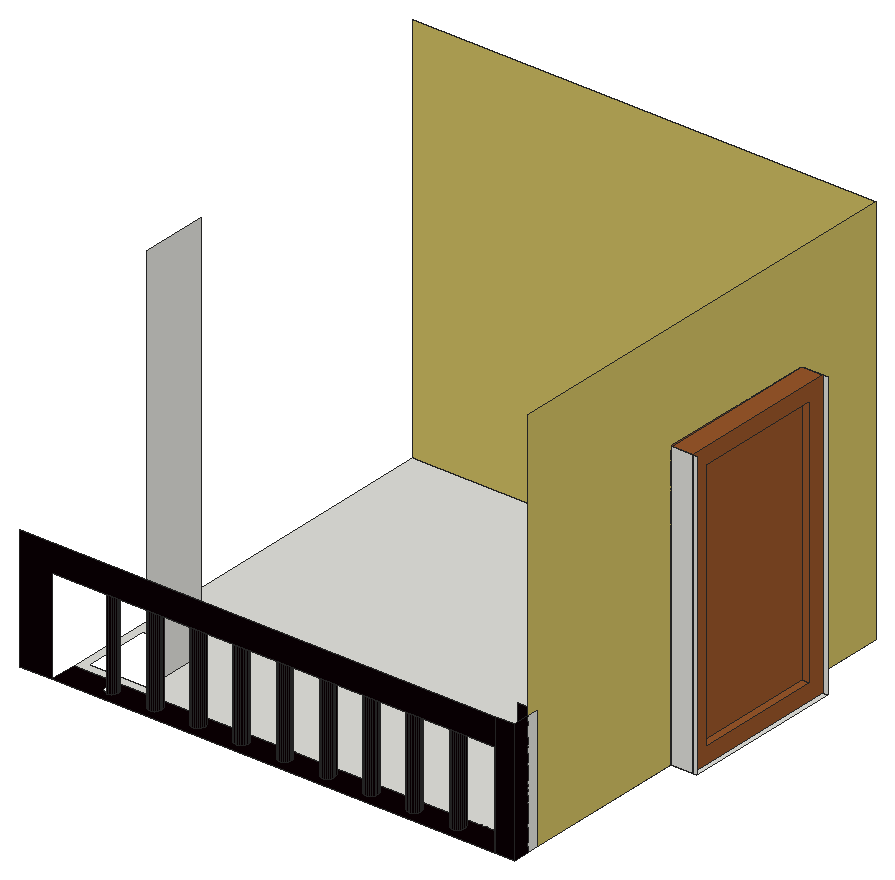
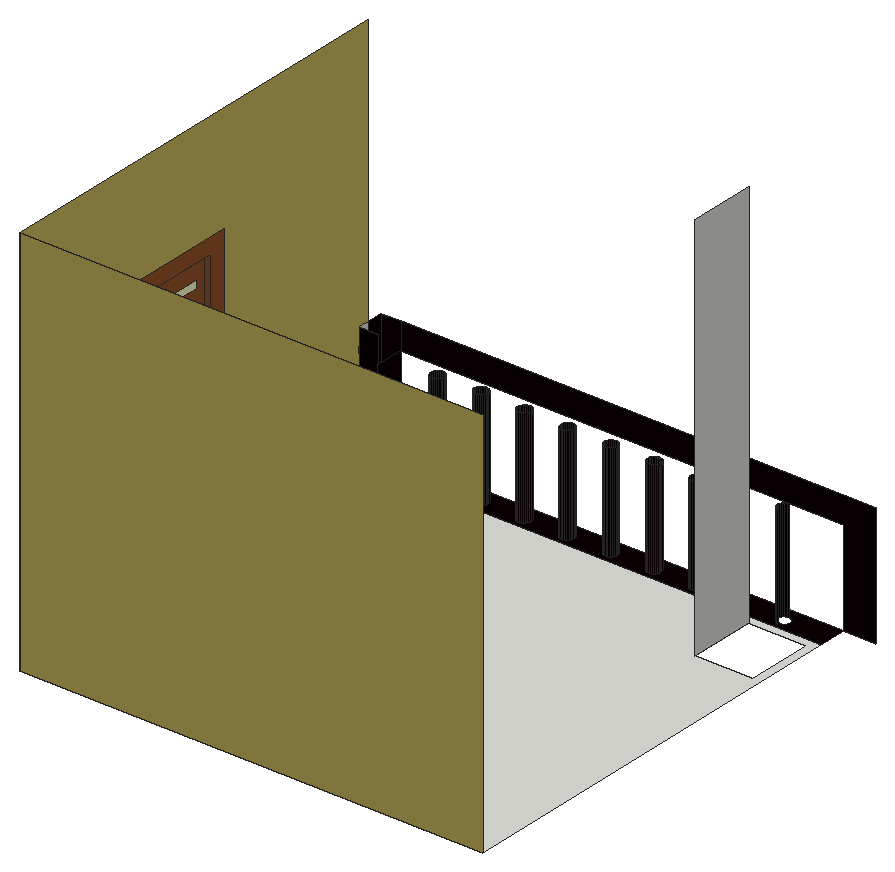
# SketchUp Ruby script. Lengths in inches.
U = 1.inch
M = Sketchup.active_model
def pt(a) = Geom::Point3d.new(a.map { |v| v * U })
def face(e, loops, mat)
  f = e.add_face(loops[0].map { |a| pt(a) })
  loops[1..].each { |l| e.add_face(l.map { |a| pt(a) }).erase! }
  f.material = f.back_material = mat if mat
  f
end
# faces: each face lists its corners as indices into pts; further lists are holes
def faces(e, pts, list, mat = nil) = list.each { |f| face(e, (f[0].is_a?(Array) ? f : [f]).map { |l| l.map { |i| pts[i] } }, mat) }
# xy, xz, yz: faces in a plane at the given z, y or x. An outline is a flat list of corners, or four numbers for a rectangle; further outlines are holes
def ring(l) = l.size == 4 ? [[l[0], l[1]], [l[2], l[1]], [l[2], l[3]], [l[0], l[3]]] : l.each_slice(2).to_a
def flat(e, list, mat, &to3) = list.each { |f| face(e, (f[0].is_a?(Array) ? f : [f]).map { |l| ring(l).map { |u, v| to3.(u, v) } }, mat) }
def xy(e, z, list, mat = nil) = flat(e, list, mat) { |x, y| [x, y, z] }
def xz(e, y, list, mat = nil) = flat(e, list, mat) { |x, z| [x, y, z] }
def yz(e, x, list, mat = nil) = flat(e, list, mat) { |y, z| [x, y, z] }
def lines(e, pts, list) = list.each { |a, b| e.add_line(pt(pts[a]), pt(pts[b])) }
# prism: a flat outline (further loops are holes) pulled along v
def prism(e, loops, v, mat = nil)
  f = face(e, loops, mat); d = Geom::Vector3d.new(v.map { |x| x * U })
  f.pushpull(f.normal.samedirection?(d) ? d.length : -d.length)
end
def box(e, o, s, mat = nil) = prism(e, [[o, [o[0] + s[0], o[1], o[2]], [o[0] + s[0], o[1] + s[1], o[2]], [o[0], o[1] + s[1], o[2]]]], [0, 0, s[2]], mat)
def at(x, y, z, deg = 0) = Geom::Transformation.translation(pt([x, y, z])) * Geom::Transformation.rotation(ORIGIN, Z_AXIS, deg.degrees)
def axes(o, x, y, z) = Geom::Transformation.new([*x, 0, *y, 0, *z, 0, *pt(o).to_a, 1])
def part(name) = M.definitions.add(name)
# library, detail: a bought-in or finely detailed component or shape, given as its bounding box
def library(name, o, s) = part(name).tap { |d| box(d.entities, o, s) }
def detail(e, o, s) = box(e.add_group.entities, o, s)
def put(e, d, t, mat = nil) = e.add_instance(d, t).tap { |i| i.material = mat if mat }
def group(e, t, mat = nil) = e.add_group.tap { |g| g.transformation = t; g.material = mat if mat }.entities
root = M.entities
M.materials.add("[Color D05]").color = [208, 191, 99]
M.materials.add("[Color E01]").color = [255, 255, 204]
M.materials.add("[Metal Seamed]").color = [11, 0, 4]
M.materials.add("[Wood Cherry Original]").color = [152, 86, 42]
c1 = part("Group\#1")
xy(c1.entities,0,[[0,0,6.3125,48]],"[Wood Cherry Original]")
xy(c1.entities,4.83,[[2.3125,4.83,3.9375,43.17]])
xy(c1.entities,4.83,[[0,4.83,2.3125,43.17],[3.9375,4.83,6.3125,43.17]],"[Wood Cherry Original]")
xy(c1.entities,79.17,[[2.3125,4.83,3.9375,43.17]])
xy(c1.entities,79.17,[[0,4.83,2.3125,43.17],[3.9375,4.83,6.3125,43.17]],"[Wood Cherry Original]")
xy(c1.entities,84,[[0,0,6.3125,48]],"[Wood Cherry Original]")
xz(c1.entities,0,[[0,0,6.3125,84]],"[Wood Cherry Original]")
xz(c1.entities,4.83,[[2.3125,4.83,3.9375,79.17]])
xz(c1.entities,4.83,[[0,4.83,2.3125,79.17],[3.9375,4.83,6.3125,79.17]],"[Wood Cherry Original]")
xz(c1.entities,43.17,[[2.3125,4.83,3.9375,79.17]])
xz(c1.entities,43.17,[[0,4.83,2.3125,79.17],[3.9375,4.83,6.3125,79.17]],"[Wood Cherry Original]")
xz(c1.entities,48,[[0,0,6.3125,84]],"[Wood Cherry Original]")
yz(c1.entities,0,[[[0,0,48,84],[4.83,4.83,43.17,79.17]]],"[Wood Cherry Original]")
yz(c1.entities,2.3125,[[7.68,9.76,40.37,11.76],[7.68,18.32,40.37,20.32],[7.68,27.01,40.37,29.01],[7.68,35.69,40.37,37.69],[7.68,44.38,40.37,46.38],
  [7.68,53.07,40.37,55.07],[7.68,61.76,40.37,63.76],[7.68,70.44,40.37,72.44]],"[Color E01]")
yz(c1.entities,2.3125,[[[4.83,4.83,43.17,79.17],[7.68,70.44,40.37,72.44],[7.68,61.76,40.37,63.76],[7.68,53.07,40.37,55.07],[7.68,44.38,40.37,46.38],[7.68,35.69,40.37,37.69],[7.68,27.01,40.37,29.01],[7.68,18.32,40.37,20.32],[7.68,9.76,40.37,11.76]]],"[Wood Cherry Original]")
yz(c1.entities,3.9375,[[4.83,4.83,43.17,79.17]],"[Wood Cherry Original]")
yz(c1.entities,6.3125,[[[0,0,48,84],[4.83,4.83,43.17,79.17]]],"[Wood Cherry Original]")
xy(root,148.4375,[[152.3,62.41,158,70.73],[48.66,65.07,48.15,65.08,47.67,65.22,47.23,65.48,46.88,65.84,46.64,66.29,46.51,66.78,46.52,67.28,46.66,67.77,46.92,68.2,47.28,68.55,47.73,68.8,48.22,68.92,48.72,68.91,49.21,68.78,49.64,68.52,50,68.15,50.24,67.71,50.36,67.22,50.36,66.71,50.22,66.23,49.96,65.79,49.59,65.44,49.15,65.2],[61.41,65.07,60.9,65.08,60.42,65.22,59.98,65.48,59.63,65.84,59.39,66.29,59.26,66.78,59.27,67.28,59.41,67.77,59.67,68.2,60.03,68.55,60.48,68.8,60.97,68.92,61.47,68.91,61.96,68.78,62.39,68.52,62.75,68.15,62.99,67.71,63.11,67.22,63.11,66.71,62.97,66.23,62.71,65.79,62.34,65.44,61.9,65.2],[74.16,65.07,73.65,65.08,73.17,65.22,72.73,65.48,72.38,65.84,72.14,66.29,72.01,66.78,72.02,67.28,72.16,67.77,72.42,68.2,72.78,68.55,73.23,68.8,73.72,68.92,74.22,68.91,74.71,68.78,75.14,68.52,75.5,68.15,75.74,67.71,75.86,67.22,75.86,66.71,75.72,66.23,75.46,65.79,75.09,65.44,74.65,65.2],[86.91,65.07,86.4,65.08,85.92,65.22,85.48,65.48,85.13,65.84,84.89,66.29,84.76,66.78,84.77,67.28,84.91,67.77,85.17,68.2,85.53,68.55,85.98,68.8,86.47,68.92,86.97,68.91,87.46,68.78,87.89,68.52,88.25,68.15,88.49,67.71,88.61,67.22,88.61,66.71,88.47,66.23,88.21,65.79,87.84,65.44,87.4,65.2],
  [99.66,65.07,99.15,65.08,98.67,65.22,98.23,65.48,97.88,65.84,97.64,66.29,97.51,66.78,97.52,67.28,97.66,67.77,97.92,68.2,98.28,68.55,98.73,68.8,99.22,68.92,99.72,68.91,100.21,68.78,100.64,68.52,101,68.15,101.24,67.71,101.36,67.22,101.36,66.71,101.22,66.23,100.96,65.79,100.59,65.44,100.15,65.2],[112.41,65.07,111.9,65.08,111.42,65.22,110.98,65.48,110.63,65.84,110.39,66.29,110.26,66.78,110.27,67.28,110.41,67.77,110.67,68.2,111.03,68.55,111.48,68.8,111.97,68.92,112.47,68.91,112.96,68.78,113.39,68.52,113.75,68.15,113.99,67.71,114.11,67.22,114.11,66.71,113.97,66.23,113.71,65.79,113.34,65.44,112.9,65.2],[125.16,65.07,124.65,65.08,124.17,65.22,123.73,65.48,123.38,65.84,123.14,66.29,123.01,66.78,123.02,67.28,123.16,67.77,123.42,68.2,123.78,68.55,124.23,68.8,124.72,68.92,125.22,68.91,125.71,68.78,126.14,68.52,126.5,68.15,126.74,67.71,126.86,67.22,126.86,66.71,126.72,66.23,126.46,65.79,126.09,65.44,125.65,65.2],[137.97,65.07,137.47,65.08,136.98,65.22,136.55,65.48,136.2,65.84,135.95,66.29,135.83,66.78,135.83,67.28,135.97,67.77,136.23,68.2,136.6,68.55,137.04,68.8,137.53,68.92,138.04,68.91,138.52,68.78,138.96,68.52,139.31,68.15,139.55,67.71,139.68,67.22,139.67,66.71,139.53,66.23,139.27,65.79,138.91,65.44,138.46,65.2],[[21.75,70.73,158,195.41],[24.07,73.08,41.19,92.83]],
  [158,120.11,165.5625,168.11]])
xy(root,148.4375,[[[21.75,62.41,152.3,70.73],[35.91,65.07,35.4,65.08,34.92,65.22,34.48,65.48,34.13,65.84,33.89,66.29,33.76,66.78,33.77,67.28,33.91,67.77,34.17,68.2,34.53,68.55,34.98,68.8,35.47,68.92,35.97,68.91,36.46,68.78,36.89,68.52,37.25,68.15,37.49,67.71,37.61,67.22,37.61,66.71,37.47,66.23,37.21,65.79,36.84,65.44,36.4,65.2],[48.66,65.07,48.15,65.08,47.67,65.22,47.23,65.48,46.88,65.84,46.64,66.29,46.51,66.78,46.52,67.28,46.66,67.77,46.92,68.2,47.28,68.55,47.73,68.8,48.22,68.92,48.72,68.91,49.21,68.78,49.64,68.52,50,68.15,50.24,67.71,50.36,67.22,50.36,66.71,50.22,66.23,49.96,65.79,49.59,65.44,49.15,65.2],[61.41,65.07,60.9,65.08,60.42,65.22,59.98,65.48,59.63,65.84,59.39,66.29,59.26,66.78,59.27,67.28,59.41,67.77,59.67,68.2,60.03,68.55,60.48,68.8,60.97,68.92,61.47,68.91,61.96,68.78,62.39,68.52,62.75,68.15,62.99,67.71,63.11,67.22,63.11,66.71,62.97,66.23,62.71,65.79,62.34,65.44,61.9,65.2],[74.16,65.07,73.65,65.08,73.17,65.22,72.73,65.48,72.38,65.84,72.14,66.29,72.01,66.78,72.02,67.28,72.16,67.77,72.42,68.2,72.78,68.55,73.23,68.8,73.72,68.92,74.22,68.91,74.71,68.78,75.14,68.52,75.5,68.15,75.74,67.71,75.86,67.22,75.86,66.71,75.72,66.23,75.46,65.79,75.09,65.44,74.65,65.2],[86.91,65.07,86.4,65.08,85.92,65.22,85.48,65.48,85.13,65.84,84.89,66.29,84.76,66.78,84.77,67.28,84.91,67.77,85.17,68.2,85.53,68.55,85.98,68.8,86.47,68.92,86.97,68.91,87.46,68.78,87.89,68.52,88.25,68.15,88.49,67.71,88.61,67.22,88.61,66.71,88.47,66.23,88.21,65.79,87.84,65.44,87.4,65.2],[99.66,65.07,99.15,65.08,98.67,65.22,98.23,65.48,97.88,65.84,97.64,66.29,97.51,66.78,97.52,67.28,97.66,67.77,97.92,68.2,98.28,68.55,98.73,68.8,99.22,68.92,99.72,68.91,100.21,68.78,100.64,68.52,101,68.15,101.24,67.71,101.36,67.22,101.36,66.71,101.22,66.23,100.96,65.79,100.59,65.44,100.15,65.2],[112.41,65.07,111.9,65.08,111.42,65.22,110.98,65.48,110.63,65.84,110.39,66.29,110.26,66.78,110.27,67.28,110.41,67.77,110.67,68.2,111.03,68.55,111.48,68.8,111.97,68.92,112.47,68.91,112.96,68.78,113.39,68.52,113.75,68.15,113.99,67.71,114.11,67.22,114.11,66.71,113.97,66.23,113.71,65.79,113.34,65.44,112.9,65.2],[125.16,65.07,124.65,65.08,124.17,65.22,123.73,65.48,123.38,65.84,123.14,66.29,123.01,66.78,123.02,67.28,123.16,67.77,123.42,68.2,123.78,68.55,124.23,68.8,124.72,68.92,125.22,68.91,125.71,68.78,126.14,68.52,126.5,68.15,126.74,67.71,126.86,67.22,126.86,66.71,126.72,66.23,126.46,65.79,126.09,65.44,125.65,65.2],[137.97,65.07,137.47,65.08,136.98,65.22,136.55,65.48,136.2,65.84,135.95,66.29,135.83,66.78,135.83,67.28,135.97,67.77,136.23,68.2,136.6,68.55,137.04,68.8,137.53,68.92,138.04,68.91,138.52,68.78,138.96,68.52,139.31,68.15,139.55,67.71,139.68,67.22,139.67,66.71,139.53,66.23,139.27,65.79,138.91,65.44,138.46,65.2]]],"[Metal Seamed]")
xz(root,62.41,[[12.3125,148.4375,21.75,148.4375,21.75,176.54,152.3,176.54,152.3,184.4375,12.3125,184.4375],[152.3,148.4375,158,184.4375]],"[Metal Seamed]")
xz(root,70.73,[[152.3,148.4375,158,184.4375]],"[Metal Seamed]")
xz(root,120.11,[[158,148.4375,165.5625,232.4375]])
xz(root,168.11,[[158,148.4375,165.5625,232.4375]])
xz(root,195.41,[[21.75,148.4375,158,264]],"[Color D05]")
yz(root,37.61,[[66.71,148.4375,67.22,178.3125]],"[Metal Seamed]")
yz(root,41.19,[[73.08,148.4375,92.83,263.5625]])
yz(root,50.36,[[66.71,148.4375,67.22,177.1875]],"[Metal Seamed]")
yz(root,63.11,[[66.71,148.4375,67.22,177]],"[Metal Seamed]")
yz(root,75.86,[[66.71,148.4375,67.22,177.125]],"[Metal Seamed]")
yz(root,88.61,[[66.71,148.4375,67.22,177.0625]],"[Metal Seamed]")
yz(root,101.36,[[66.71,148.4375,67.22,177.1875]],"[Metal Seamed]")
yz(root,114.11,[[66.71,148.4375,67.22,177.3125]],"[Metal Seamed]")
yz(root,126.86,[[66.71,148.4375,67.22,177.75]],"[Metal Seamed]")
yz(root,135.83,[[66.78,148.4375,67.28,177.4375]],"[Metal Seamed]")
yz(root,152.3,[[62.41,148.4375,70.73,176.54]],"[Metal Seamed]")
yz(root,158,[[67.28,148.4375,70.73,184.4375]])
yz(root,158,[[70.73,148.4375,70.73,184.4375,67.28,184.4375,67.28,264,195.41,264,195.41,148.4375,168.11,148.4375,168.11,232.4375,120.11,232.4375,120.11,148.4375]],"[Color D05]")
yz(root,158,[[62.41,148.4375,67.28,184.4375]],"[Metal Seamed]")
p = [[35.91,65.07,148.4375],[36.4,65.2,148.4375],[36.4,65.2,178.3125],[35.91,65.07,178.3125],[47.67,65.22,148.4375],[48.15,65.08,148.4375],
  [48.15,65.08,177.1875],[47.67,65.22,177.1875],[48.66,65.07,148.4375],[48.66,65.07,177.1875],[49.15,65.2,148.4375],[49.15,65.2,177.1875],
  [60.42,65.22,148.4375],[60.9,65.08,148.4375],[60.9,65.08,177],[60.42,65.22,177],[61.41,65.07,148.4375],[61.41,65.07,177],
  [61.9,65.2,148.4375],[61.9,65.2,177],[73.17,65.22,148.4375],[73.65,65.08,148.4375],[73.65,65.08,177.125],[73.17,65.22,177.125],
  [74.16,65.07,148.4375],[74.16,65.07,177.125],[74.65,65.2,148.4375],[74.65,65.2,177.125],[85.92,65.22,148.4375],[86.4,65.08,148.4375],
  [86.4,65.08,177.0625],[85.92,65.22,177.0625],[86.91,65.07,148.4375],[86.91,65.07,177.0625],[87.4,65.2,148.4375],[87.4,65.2,177.0625],
  [98.67,65.22,148.4375],[99.15,65.08,148.4375],[99.15,65.08,177.1875],[98.67,65.22,177.1875],[99.66,65.07,148.4375],[99.66,65.07,177.1875],
  [100.15,65.2,148.4375],[100.15,65.2,177.1875],[111.42,65.22,148.4375],[111.9,65.08,148.4375],[111.9,65.08,177.3125],[111.42,65.22,177.3125],
  [112.41,65.07,148.4375],[112.41,65.07,177.3125],[112.9,65.2,148.4375],[112.9,65.2,177.3125],[124.17,65.22,148.4375],[124.65,65.08,148.4375],
  [124.65,65.08,177.75],[124.17,65.22,177.75],[125.16,65.07,148.4375],[125.16,65.07,177.75],[125.65,65.2,148.4375],[125.65,65.2,177.75],
  [136.98,65.22,148.4375],[137.47,65.08,148.4375],[137.47,65.08,177.4375],[136.98,65.22,177.4375],[137.97,65.07,148.4375],[137.97,65.07,177.4375],
  [138.46,65.2,148.4375],[138.46,65.2,177.4375],[36.84,65.44,148.4375],[36.84,65.44,178.3125],[47.23,65.48,148.4375],[47.23,65.48,177.1875],
  [49.59,65.44,148.4375],[49.59,65.44,177.1875],[59.98,65.48,148.4375],[59.98,65.48,177],[62.34,65.44,148.4375],[62.34,65.44,177],
  [72.73,65.48,148.4375],[72.73,65.48,177.125],[75.09,65.44,148.4375],[75.09,65.44,177.125],[85.48,65.48,148.4375],[85.48,65.48,177.0625],
  [87.84,65.44,148.4375],[87.84,65.44,177.0625],[98.23,65.48,148.4375],[98.23,65.48,177.1875],[100.59,65.44,148.4375],[100.59,65.44,177.1875],
  [110.98,65.48,148.4375],[110.98,65.48,177.3125],[113.34,65.44,148.4375],[113.34,65.44,177.3125],[123.73,65.48,148.4375],[123.73,65.48,177.75],
  [126.09,65.44,148.4375],[126.09,65.44,177.75],[136.55,65.48,148.4375],[136.55,65.48,177.4375],[138.91,65.44,148.4375],[138.91,65.44,177.4375],
  [37.21,65.79,148.4375],[37.21,65.79,178.3125],[49.96,65.79,148.4375],[49.96,65.79,177.1875],[62.71,65.79,148.4375],[62.71,65.79,177],
  [75.46,65.79,148.4375],[75.46,65.79,177.125],[88.21,65.79,148.4375],[88.21,65.79,177.0625],[100.96,65.79,148.4375],[100.96,65.79,177.1875],
  [113.71,65.79,148.4375],[113.71,65.79,177.3125],[126.46,65.79,148.4375],[126.46,65.79,177.75],[139.27,65.79,148.4375],[139.27,65.79,177.4375],
  [46.88,65.84,148.4375],[46.88,65.84,177.1875],[59.63,65.84,148.4375],[59.63,65.84,177],[72.38,65.84,148.4375],[72.38,65.84,177.125],
  [85.13,65.84,148.4375],[85.13,65.84,177.0625],[97.88,65.84,148.4375],[97.88,65.84,177.1875],[110.63,65.84,148.4375],[110.63,65.84,177.3125],
  [123.38,65.84,148.4375],[123.38,65.84,177.75],[136.2,65.84,148.4375],[136.2,65.84,177.4375],[37.47,66.23,148.4375],[37.47,66.23,178.3125],
  [46.64,66.29,148.4375],[46.64,66.29,177.1875],[50.22,66.23,148.4375],[50.22,66.23,177.1875],[59.39,66.29,148.4375],[59.39,66.29,177],
  [62.97,66.23,148.4375],[62.97,66.23,177],[72.14,66.29,148.4375],[72.14,66.29,177.125],[75.72,66.23,148.4375],[75.72,66.23,177.125],
  [84.89,66.29,148.4375],[84.89,66.29,177.0625],[88.47,66.23,148.4375],[88.47,66.23,177.0625],[97.64,66.29,148.4375],[97.64,66.29,177.1875],
  [101.22,66.23,148.4375],[101.22,66.23,177.1875],[110.39,66.29,148.4375],[110.39,66.29,177.3125],[113.97,66.23,148.4375],[113.97,66.23,177.3125],
  [123.14,66.29,148.4375],[123.14,66.29,177.75],[126.72,66.23,148.4375],[126.72,66.23,177.75],[135.95,66.29,148.4375],[135.95,66.29,177.4375],
  [139.53,66.23,148.4375],[139.53,66.23,177.4375],[37.61,66.71,148.4375],[37.61,66.71,178.3125],[50.36,66.71,148.4375],[50.36,66.71,177.1875],
  [63.11,66.71,148.4375],[63.11,66.71,177],[75.86,66.71,148.4375],[75.86,66.71,177.125],[88.61,66.71,148.4375],[88.61,66.71,177.0625],
  [101.36,66.71,148.4375],[101.36,66.71,177.1875],[114.11,66.71,148.4375],[114.11,66.71,177.3125],[126.86,66.71,148.4375],[126.86,66.71,177.75],
  [139.67,66.71,148.4375],[139.67,66.71,177.4375],[46.51,66.78,148.4375],[46.51,66.78,177.1875],[59.26,66.78,148.4375],[59.26,66.78,177],
  [72.01,66.78,148.4375],[72.01,66.78,177.125],[84.76,66.78,148.4375],[84.76,66.78,177.0625],[97.51,66.78,148.4375],[97.51,66.78,177.1875],
  [110.26,66.78,148.4375],[110.26,66.78,177.3125],[123.01,66.78,148.4375],[123.01,66.78,177.75],[135.83,66.78,148.4375],[135.83,66.78,177.4375],
  [139.68,67.22,148.4375],[139.68,67.22,177.4375],[46.52,67.28,148.4375],[46.52,67.28,177.1875],[59.27,67.28,148.4375],[59.27,67.28,177],
  [72.02,67.28,148.4375],[72.02,67.28,177.125],[84.77,67.28,148.4375],[84.77,67.28,177.0625],[97.52,67.28,148.4375],[97.52,67.28,177.1875],
  [110.27,67.28,148.4375],[110.27,67.28,177.3125],[123.02,67.28,148.4375],[123.02,67.28,177.75],[37.61,67.22,148.4375],[37.49,67.71,148.4375],
  [37.49,67.71,178.3125],[37.61,67.22,178.3125],[50.36,67.22,148.4375],[50.24,67.71,148.4375],[50.24,67.71,177.1875],[50.36,67.22,177.1875],
  [63.11,67.22,148.4375],[62.99,67.71,148.4375],[62.99,67.71,177],[63.11,67.22,177],[75.86,67.22,148.4375],[75.74,67.71,148.4375],
  [75.74,67.71,177.125],[75.86,67.22,177.125],[88.61,67.22,148.4375],[88.49,67.71,148.4375],[88.49,67.71,177.0625],[88.61,67.22,177.0625],
  [101.36,67.22,148.4375],[101.24,67.71,148.4375],[101.24,67.71,177.1875],[101.36,67.22,177.1875],[114.11,67.22,148.4375],[113.99,67.71,148.4375],
  [113.99,67.71,177.3125],[114.11,67.22,177.3125],[126.86,67.22,148.4375],[126.74,67.71,148.4375],[126.74,67.71,177.75],[126.86,67.22,177.75],
  [139.55,67.71,148.4375],[139.55,67.71,177.4375],[46.66,67.77,148.4375],[46.66,67.77,177.1875],[59.41,67.77,148.4375],[59.41,67.77,177],
  [72.16,67.77,148.4375],[72.16,67.77,177.125],[84.91,67.77,148.4375],[84.91,67.77,177.0625],[97.66,67.77,148.4375],[97.66,67.77,177.1875],
  [110.41,67.77,148.4375],[110.41,67.77,177.3125],[123.16,67.77,148.4375],[123.16,67.77,177.75],[135.97,67.77,148.4375],[135.83,67.28,148.4375],
  [135.83,67.28,177.4375],[135.97,67.77,177.4375],[37.25,68.15,148.4375],[37.25,68.15,178.3125],[50,68.15,148.4375],[50,68.15,177.1875],
  [62.75,68.15,148.4375],[62.75,68.15,177],[75.5,68.15,148.4375],[75.5,68.15,177.125],[88.25,68.15,148.4375],[88.25,68.15,177.0625],
  [101,68.15,148.4375],[101,68.15,177.1875],[113.75,68.15,148.4375],[113.75,68.15,177.3125],[126.5,68.15,148.4375],[126.5,68.15,177.75],
  [139.31,68.15,148.4375],[139.31,68.15,177.4375],[46.92,68.2,148.4375],[46.92,68.2,177.1875],[59.67,68.2,148.4375],[59.67,68.2,177],
  [72.42,68.2,148.4375],[72.42,68.2,177.125],[85.17,68.2,148.4375],[85.17,68.2,177.0625],[97.92,68.2,148.4375],[97.92,68.2,177.1875],
  [110.67,68.2,148.4375],[110.67,68.2,177.3125],[123.42,68.2,148.4375],[123.42,68.2,177.75],[136.23,68.2,148.4375],[136.23,68.2,177.4375],
  [36.89,68.52,148.4375],[36.89,68.52,178.3125],[47.28,68.55,148.4375],[47.28,68.55,177.1875],[49.64,68.52,148.4375],[49.64,68.52,177.1875],
  [60.03,68.55,148.4375],[60.03,68.55,177],[62.39,68.52,148.4375],[62.39,68.52,177],[72.78,68.55,148.4375],[72.78,68.55,177.125],
  [75.14,68.52,148.4375],[75.14,68.52,177.125],[85.53,68.55,148.4375],[85.53,68.55,177.0625],[87.89,68.52,148.4375],[87.89,68.52,177.0625],
  [98.28,68.55,148.4375],[98.28,68.55,177.1875],[100.64,68.52,148.4375],[100.64,68.52,177.1875],[111.03,68.55,148.4375],[111.03,68.55,177.3125],
  [113.39,68.52,148.4375],[113.39,68.52,177.3125],[123.78,68.55,148.4375],[123.78,68.55,177.75],[126.14,68.52,148.4375],[126.14,68.52,177.75],
  [136.6,68.55,148.4375],[136.6,68.55,177.4375],[138.96,68.52,148.4375],[138.96,68.52,177.4375],[36.46,68.78,148.4375],[36.46,68.78,178.3125],
  [49.21,68.78,148.4375],[49.21,68.78,177.1875],[61.96,68.78,148.4375],[61.96,68.78,177],[74.71,68.78,148.4375],[74.71,68.78,177.125],
  [87.46,68.78,148.4375],[87.46,68.78,177.0625],[100.21,68.78,148.4375],[100.21,68.78,177.1875],[112.96,68.78,148.4375],[112.96,68.78,177.3125],
  [125.71,68.78,148.4375],[125.71,68.78,177.75],[138.52,68.78,148.4375],[138.52,68.78,177.4375],[47.73,68.8,148.4375],[47.73,68.8,177.1875],
  [60.48,68.8,148.4375],[60.48,68.8,177],[73.23,68.8,148.4375],[73.23,68.8,177.125],[85.98,68.8,148.4375],[85.98,68.8,177.0625],
  [98.73,68.8,148.4375],[98.73,68.8,177.1875],[111.48,68.8,148.4375],[111.48,68.8,177.3125],[124.23,68.8,148.4375],[124.23,68.8,177.75],
  [137.04,68.8,148.4375],[137.04,68.8,177.4375],[35.97,68.91,148.4375],[35.97,68.91,178.3125],[48.22,68.92,148.4375],[48.22,68.92,177.1875],
  [48.72,68.91,148.4375],[48.72,68.91,177.1875],[60.97,68.92,148.4375],[60.97,68.92,177],[61.47,68.91,148.4375],[61.47,68.91,177],
  [73.72,68.92,148.4375],[73.72,68.92,177.125],[74.22,68.91,148.4375],[74.22,68.91,177.125],[86.47,68.92,148.4375],[86.47,68.92,177.0625],
  [86.97,68.91,148.4375],[86.97,68.91,177.0625],[99.22,68.92,148.4375],[99.22,68.92,177.1875],[99.72,68.91,148.4375],[99.72,68.91,177.1875],
  [111.97,68.92,148.4375],[111.97,68.92,177.3125],[112.47,68.91,148.4375],[112.47,68.91,177.3125],[124.72,68.92,148.4375],[124.72,68.92,177.75],
  [125.22,68.91,148.4375],[125.22,68.91,177.75],[137.53,68.92,148.4375],[137.53,68.92,177.4375],[138.04,68.91,148.4375],[138.04,68.91,177.4375]]
faces(root,p,[[0,1,2,3],[4,5,6,7],[5,8,9,6],[8,10,11,9],[12,13,14,15],[13,16,17,14],[16,18,19,17],[20,21,22,23],
  [21,24,25,22],[24,26,27,25],[28,29,30,31],[29,32,33,30],[32,34,35,33],[36,37,38,39],[37,40,41,38],[40,42,43,41],
  [44,45,46,47],[45,48,49,46],[48,50,51,49],[52,53,54,55],[53,56,57,54],[56,58,59,57],[60,61,62,63],[61,64,65,62],
  [64,66,67,65],[1,68,69,2],[70,4,7,71],[10,72,73,11],[74,12,15,75],[18,76,77,19],[78,20,23,79],[26,80,81,27],
  [82,28,31,83],[34,84,85,35],[86,36,39,87],[42,88,89,43],[90,44,47,91],[50,92,93,51],[94,52,55,95],[58,96,97,59],
  [98,60,63,99],[66,100,101,67],[68,102,103,69],[72,104,105,73],[76,106,107,77],[80,108,109,81],[84,110,111,85],[88,112,113,89],
  [92,114,115,93],[96,116,117,97],[100,118,119,101],[120,70,71,121],[122,74,75,123],[124,78,79,125],[126,82,83,127],[128,86,87,129],
  [130,90,91,131],[132,94,95,133],[134,98,99,135],[102,136,137,103],[138,120,121,139],[104,140,141,105],[142,122,123,143],[106,144,145,107],
  [146,124,125,147],[108,148,149,109],[150,126,127,151],[110,152,153,111],[154,128,129,155],[112,156,157,113],[158,130,131,159],[114,160,161,115],
  [162,132,133,163],[116,164,165,117],[166,134,135,167],[118,168,169,119],[136,170,171,137],[140,172,173,141],[144,174,175,145],[148,176,177,149],
  [152,178,179,153],[156,180,181,157],[160,182,183,161],[164,184,185,165],[168,186,187,169],[188,138,139,189],[190,142,143,191],[192,146,147,193],
  [194,150,151,195],[196,154,155,197],[198,158,159,199],[200,162,163,201],[202,166,167,203],[186,204,205,187],[206,188,189,207],[208,190,191,209],
  [210,192,193,211],[212,194,195,213],[214,196,197,215],[216,198,199,217],[218,200,201,219],[220,221,222,223],[224,225,226,227],[228,229,230,231],
  [232,233,234,235],[236,237,238,239],[240,241,242,243],[244,245,246,247],[248,249,250,251],[204,252,253,205],[254,206,207,255],[256,208,209,257],
  [258,210,211,259],[260,212,213,261],[262,214,215,263],[264,216,217,265],[266,218,219,267],[268,269,270,271],[221,272,273,222],[225,274,275,226],
  [229,276,277,230],[233,278,279,234],[237,280,281,238],[241,282,283,242],[245,284,285,246],[249,286,287,250],[252,288,289,253],[290,254,255,291],
  [292,256,257,293],[294,258,259,295],[296,260,261,297],[298,262,263,299],[300,264,265,301],[302,266,267,303],[304,268,271,305],[272,306,307,273],
  [308,290,291,309],[274,310,311,275],[312,292,293,313],[276,314,315,277],[316,294,295,317],[278,318,319,279],[320,296,297,321],[280,322,323,281],
  [324,298,299,325],[282,326,327,283],[328,300,301,329],[284,330,331,285],[332,302,303,333],[286,334,335,287],[336,304,305,337],[288,338,339,289],
  [306,340,341,307],[310,342,343,311],[314,344,345,315],[318,346,347,319],[322,348,349,323],[326,350,351,327],[330,352,353,331],[334,354,355,335],
  [338,356,357,339],[358,308,309,359],[360,312,313,361],[362,316,317,363],[364,320,321,365],[366,324,325,367],[368,328,329,369],[370,332,333,371],
  [372,336,337,373],[340,374,375,341],[376,358,359,377],[342,378,379,343],[380,360,361,381],[344,382,383,345],[384,362,363,385],[346,386,387,347],
  [388,364,365,389],[348,390,391,349],[392,366,367,393],[350,394,395,351],[396,368,369,397],[352,398,399,353],[400,370,371,401],[354,402,403,355],
  [404,372,373,405],[356,406,407,357],[378,376,377,379],[382,380,381,383],[386,384,385,387],[390,388,389,391],[394,392,393,395],[398,396,397,399],
  [402,400,401,403],[406,404,405,407]],"[Metal Seamed]")
put(root,c1,at(158,120.11,148.4375))
